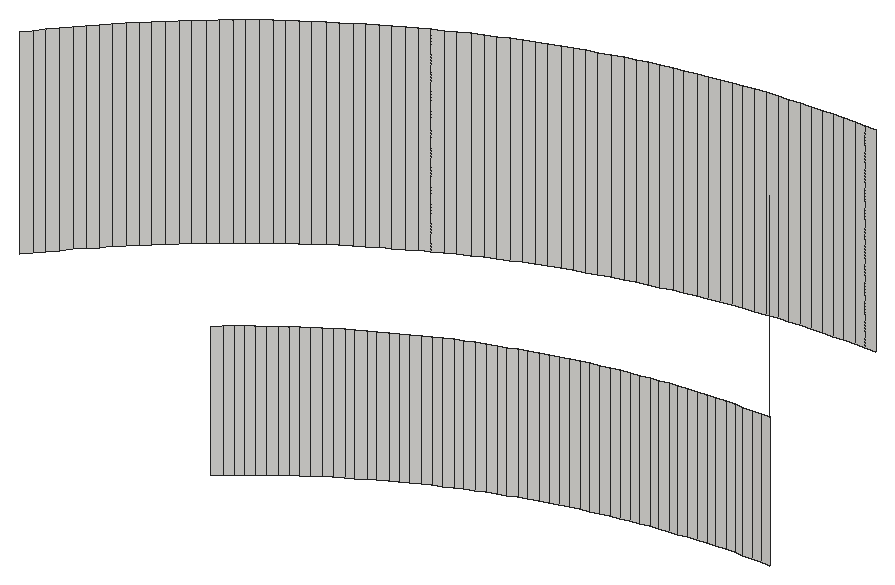
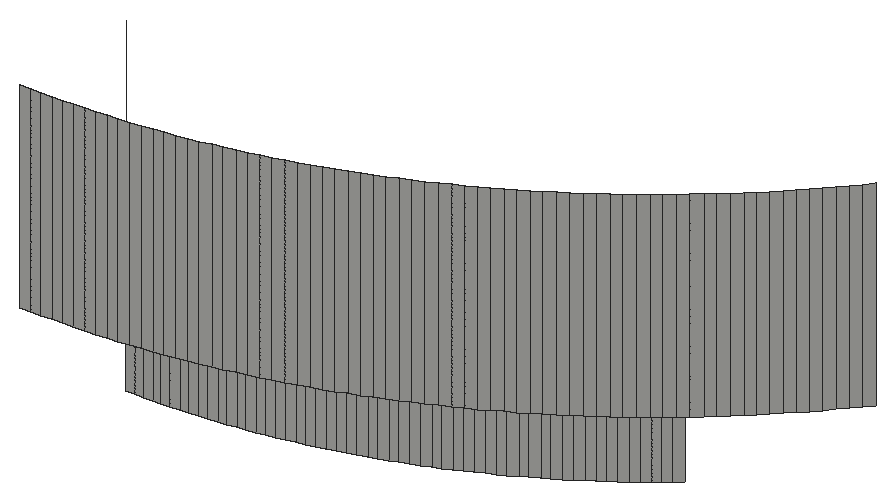
# SketchUp Ruby script. Lengths in inches.
U = 1.inch
M = Sketchup.active_model
def pt(a) = Geom::Point3d.new(a.map { |v| v * U })
def face(e, loops, mat)
  f = e.add_face(loops[0].map { |a| pt(a) })
  loops[1..].each { |l| e.add_face(l.map { |a| pt(a) }).erase! }
  f.material = f.back_material = mat if mat
  f
end
# faces: each face lists its corners as indices into pts; further lists are holes
def faces(e, pts, list, mat = nil) = list.each { |f| face(e, (f[0].is_a?(Array) ? f : [f]).map { |l| l.map { |i| pts[i] } }, mat) }
# xy, xz, yz: faces in a plane at the given z, y or x. An outline is a flat list of corners, or four numbers for a rectangle; further outlines are holes
def ring(l) = l.size == 4 ? [[l[0], l[1]], [l[2], l[1]], [l[2], l[3]], [l[0], l[3]]] : l.each_slice(2).to_a
def flat(e, list, mat, &to3) = list.each { |f| face(e, (f[0].is_a?(Array) ? f : [f]).map { |l| ring(l).map { |u, v| to3.(u, v) } }, mat) }
def xy(e, z, list, mat = nil) = flat(e, list, mat) { |x, y| [x, y, z] }
def xz(e, y, list, mat = nil) = flat(e, list, mat) { |x, z| [x, y, z] }
def yz(e, x, list, mat = nil) = flat(e, list, mat) { |y, z| [x, y, z] }
def lines(e, pts, list) = list.each { |a, b| e.add_line(pt(pts[a]), pt(pts[b])) }
# prism: a flat outline (further loops are holes) pulled along v
def prism(e, loops, v, mat = nil)
  f = face(e, loops, mat); d = Geom::Vector3d.new(v.map { |x| x * U })
  f.pushpull(f.normal.samedirection?(d) ? d.length : -d.length)
end
def box(e, o, s, mat = nil) = prism(e, [[o, [o[0] + s[0], o[1], o[2]], [o[0] + s[0], o[1] + s[1], o[2]], [o[0], o[1] + s[1], o[2]]]], [0, 0, s[2]], mat)
def at(x, y, z, deg = 0) = Geom::Transformation.translation(pt([x, y, z])) * Geom::Transformation.rotation(ORIGIN, Z_AXIS, deg.degrees)
def axes(o, x, y, z) = Geom::Transformation.new([*x, 0, *y, 0, *z, 0, *pt(o).to_a, 1])
def part(name) = M.definitions.add(name)
# library, detail: a bought-in or finely detailed component or shape, given as its bounding box
def library(name, o, s) = part(name).tap { |d| box(d.entities, o, s) }
def detail(e, o, s) = box(e.add_group.entities, o, s)
def put(e, d, t, mat = nil) = e.add_instance(d, t).tap { |i| i.material = mat if mat }
def group(e, t, mat = nil) = e.add_group.tap { |g| g.transformation = t; g.material = mat if mat }.entities
root = M.entities
M.materials.add("[Formica Graystone]").color = [224, 223, 219]
xz(root,441.99,[[17.48,422.82,17.61,424.82]],"[Formica Graystone]")
xz(root,442,[[17.74,422.82,17.87,424.82],[17.87,422.82,18,424.82]],"[Formica Graystone]")
xz(root,444,[[17.6875,424.82,17.84,427.82],[17.84,424.82,18,427.82]],"[Formica Graystone]")
p = [[11.51,439.6,422.82],[11.51,439.6,424.82],[11.61,439.6875,424.82],[11.61,439.6875,422.82],[11.71,439.77,424.82],[11.71,439.77,422.82],
  [11.81,439.85,424.82],[11.81,439.85,422.82],[11.91,439.93,424.82],[11.91,439.93,422.82],[12.02,440.01,424.82],[12.02,440.01,422.82],
  [12.12,440.09,424.82],[12.12,440.09,422.82],[12.23,440.17,424.82],[12.23,440.17,422.82],[12.34,440.24,424.82],[12.34,440.24,422.82],
  [12.44,440.31,424.82],[12.44,440.31,422.82],[12.55,440.39,424.82],[12.55,440.39,422.82],[12.66,440.46,424.82],[12.66,440.46,422.82],
  [12.78,440.53,424.82],[12.78,440.53,422.82],[12.89,440.59,424.82],[12.89,440.59,422.82],[13,440.66,424.82],[13,440.66,422.82],
  [13.11,440.72,424.82],[13.11,440.72,422.82],[13.23,440.79,424.82],[13.23,440.79,422.82],[13.34,440.85,424.82],[13.34,440.85,422.82],
  [13.46,440.91,424.82],[13.46,440.91,422.82],[13.58,440.97,424.82],[13.58,440.97,422.82],[13.69,441.03,424.82],[13.69,441.03,422.82],
  [13.8125,441.08,424.82],[13.8125,441.08,422.82],[13.93,441.14,424.82],[13.93,441.14,422.82],[14.05,441.1875,424.82],[14.05,441.1875,422.82],
  [14.17,441.24,424.82],[14.17,441.24,422.82],[14.29,441.29,424.82],[14.29,441.29,422.82],[14.42,441.34,424.82],[14.42,441.34,422.82],
  [14.54,441.38,424.82],[14.54,441.38,422.82],[14.66,441.43,424.82],[14.66,441.43,422.82],[14.79,441.47,424.82],[14.79,441.47,422.82],
  [14.91,441.51,424.82],[14.91,441.51,422.82],[15.03,441.55,424.82],[15.03,441.55,422.82],[15.16,441.59,424.82],[15.16,441.59,422.82],
  [15.29,441.625,424.82],[15.29,441.625,422.82],[15.41,441.66,424.82],[15.41,441.66,422.82],[15.54,441.69,424.82],[15.54,441.69,422.82],
  [15.67,441.72,424.82],[15.67,441.72,422.82],[15.79,441.75,424.82],[15.79,441.75,422.82],[15.92,441.78,424.82],[15.92,441.78,422.82],
  [16.05,441.81,424.82],[16.05,441.81,422.82],[16.18,441.83,424.82],[16.18,441.83,422.82],[16.31,441.86,424.82],[16.31,441.86,422.82],
  [16.4375,441.875,424.82],[16.4375,441.875,422.82],[16.57,441.9,424.82],[16.57,441.9,422.82],[16.69,441.91,424.82],[16.69,441.91,422.82],
  [16.82,441.93,424.82],[16.82,441.93,422.82],[16.95,441.95,424.82],[16.95,441.95,422.82],[17.08,441.96,424.82],[17.08,441.96,422.82],
  [17.22,441.97,424.82],[17.22,441.97,422.82],[17.35,441.98,424.82],[17.35,441.98,422.82],[17.48,441.99,424.82],[17.48,441.99,422.82],
  [17.61,441.99,422.82],[17.61,441.99,424.82],[17.74,442,424.82],[17.74,442,422.82],[8.77,439.67,424.82],[8.67,439.55,424.82],
  [8.67,439.55,427.82],[8.77,439.67,427.82],[8.875,439.79,424.82],[8.875,439.79,427.82],[8.98,439.91,424.82],[8.98,439.91,427.82],
  [9.08,440.03,424.82],[9.08,440.03,427.82],[9.1875,440.15,424.82],[9.1875,440.15,427.82],[9.3,440.26,424.82],[9.3,440.26,427.82],
  [9.4,440.375,424.82],[9.4,440.375,427.82],[9.51,440.49,424.82],[9.51,440.49,427.82],[9.625,440.6,424.82],[9.625,440.6,427.82],
  [9.74,440.7,424.82],[9.74,440.7,427.82],[9.85,440.8125,424.82],[9.85,440.8125,427.82],[9.97,440.92,424.82],[9.97,440.92,427.82],
  [10.09,441.02,424.82],[10.09,441.02,427.82],[10.21,441.125,424.82],[10.21,441.125,427.82],[10.33,441.23,424.82],[10.33,441.23,427.82],
  [10.45,441.33,424.82],[10.45,441.33,427.82],[10.57,441.42,424.82],[10.57,441.42,427.82],[10.69,441.52,424.82],[10.69,441.52,427.82],
  [10.82,441.62,424.82],[10.82,441.62,427.82],[10.95,441.71,424.82],[10.95,441.71,427.82],[11.07,441.8,424.82],[11.07,441.8,427.82],
  [11.2,441.89,424.82],[11.2,441.89,427.82],[11.33,441.98,424.82],[11.33,441.98,427.82],[11.46,442.0625,424.82],[11.46,442.0625,427.82],
  [11.6,442.15,424.82],[11.6,442.15,427.82],[11.73,442.23,424.82],[11.73,442.23,427.82],[11.86,442.3125,424.82],[11.86,442.3125,427.82],
  [12,442.39,424.82],[12,442.39,427.82],[12.14,442.47,424.82],[12.14,442.47,427.82],[12.27,442.55,424.82],[12.27,442.55,427.82],
  [12.41,442.62,424.82],[12.41,442.62,427.82],[12.55,442.69,424.82],[12.55,442.69,427.82],[12.69,442.76,424.82],[12.69,442.76,427.82],
  [12.83,442.83,424.82],[12.83,442.83,427.82],[12.98,442.9,424.82],[12.98,442.9,427.82],[13.12,442.96,424.82],[13.12,442.96,427.82],
  [13.26,443.03,424.82],[13.26,443.03,427.82],[13.41,443.09,424.82],[13.41,443.09,427.82],[13.55,443.15,424.82],[13.55,443.15,427.82],
  [13.7,443.2,424.82],[13.7,443.2,427.82],[13.85,443.26,424.82],[13.85,443.26,427.82],[13.99,443.3125,424.82],[13.99,443.3125,427.82],
  [14.14,443.36,424.82],[14.14,443.36,427.82],[14.29,443.41,424.82],[14.29,443.41,427.82],[14.44,443.46,424.82],[14.44,443.46,427.82],
  [14.59,443.51,424.82],[14.59,443.51,427.82],[14.74,443.55,424.82],[14.74,443.55,427.82],[14.89,443.59,424.82],[14.89,443.59,427.82],
  [15.05,443.63,424.82],[15.05,443.63,427.82],[15.2,443.67,424.82],[15.2,443.67,427.82],[15.35,443.7,424.82],[15.35,443.7,427.82],
  [15.51,443.74,424.82],[15.51,443.74,427.82],[15.66,443.77,424.82],[15.66,443.77,427.82],[15.8125,443.8,424.82],[15.8125,443.8,427.82],
  [15.97,443.83,424.82],[15.97,443.83,427.82],[16.12,443.85,424.82],[16.12,443.85,427.82],[16.28,443.875,424.82],[16.28,443.875,427.82],
  [16.43,443.9,424.82],[16.43,443.9,427.82],[16.59,443.92,424.82],[16.59,443.92,427.82],[16.75,443.93,424.82],[16.75,443.93,427.82],
  [16.9,443.95,424.82],[16.9,443.95,427.82],[17.06,443.96,424.82],[17.06,443.96,427.82],[17.22,443.97,424.82],[17.22,443.97,427.82],
  [17.37,443.98,424.82],[17.37,443.98,427.82],[17.53,443.99,424.82],[17.53,443.99,427.82],[17.6875,444,424.82],[17.6875,444,427.82],
  [18,442,424.82],[18,442,427.82]]
faces(root,p,[[0,1,2,3],[3,2,4,5],[5,4,6,7],[7,6,8,9],[9,8,10,11],[11,10,12,13],[13,12,14,15],[15,14,16,17],
  [17,16,18,19],[19,18,20,21],[21,20,22,23],[23,22,24,25],[25,24,26,27],[27,26,28,29],[29,28,30,31],[31,30,32,33],
  [33,32,34,35],[35,34,36,37],[37,36,38,39],[39,38,40,41],[41,40,42,43],[43,42,44,45],[45,44,46,47],[47,46,48,49],
  [49,48,50,51],[51,50,52,53],[53,52,54,55],[55,54,56,57],[57,56,58,59],[59,58,60,61],[61,60,62,63],[63,62,64,65],
  [65,64,66,67],[67,66,68,69],[69,68,70,71],[71,70,72,73],[73,72,74,75],[75,74,76,77],[77,76,78,79],[79,78,80,81],
  [81,80,82,83],[83,82,84,85],[85,84,86,87],[87,86,88,89],[89,88,90,91],[91,90,92,93],[93,92,94,95],[95,94,96,97],
  [97,96,98,99],[99,98,100,101],[102,103,104,105],[106,107,108,109],[110,106,109,111],[112,110,111,113],[114,112,113,115],[116,114,115,117],
  [118,116,117,119],[120,118,119,121],[122,120,121,123],[124,122,123,125],[126,124,125,127],[128,126,127,129],[130,128,129,131],[132,130,131,133],
  [134,132,133,135],[136,134,135,137],[138,136,137,139],[140,138,139,141],[142,140,141,143],[144,142,143,145],[146,144,145,147],[148,146,147,149],
  [150,148,149,151],[152,150,151,153],[154,152,153,155],[156,154,155,157],[158,156,157,159],[160,158,159,161],[162,160,161,163],[164,162,163,165],
  [166,164,165,167],[168,166,167,169],[170,168,169,171],[172,170,171,173],[174,172,173,175],[176,174,175,177],[178,176,177,179],[180,178,179,181],
  [182,180,181,183],[184,182,183,185],[186,184,185,187],[188,186,187,189],[190,188,189,191],[192,190,191,193],[194,192,193,195],[196,194,195,197],
  [198,196,197,199],[200,198,199,201],[202,200,201,203],[204,202,203,205],[206,204,205,207],[208,206,207,209],[210,208,209,211],[212,210,211,213],
  [214,212,213,215],[216,214,215,217],[218,216,217,219],[220,218,219,221],[222,220,221,223],[224,222,223,225],[226,224,225,227],[228,226,227,229],
  [230,228,229,231],[232,230,231,233],[234,232,233,235],[236,234,235,237],[238,236,237,239]],"[Formica Graystone]")
lines(root,p,[[240,241]])
